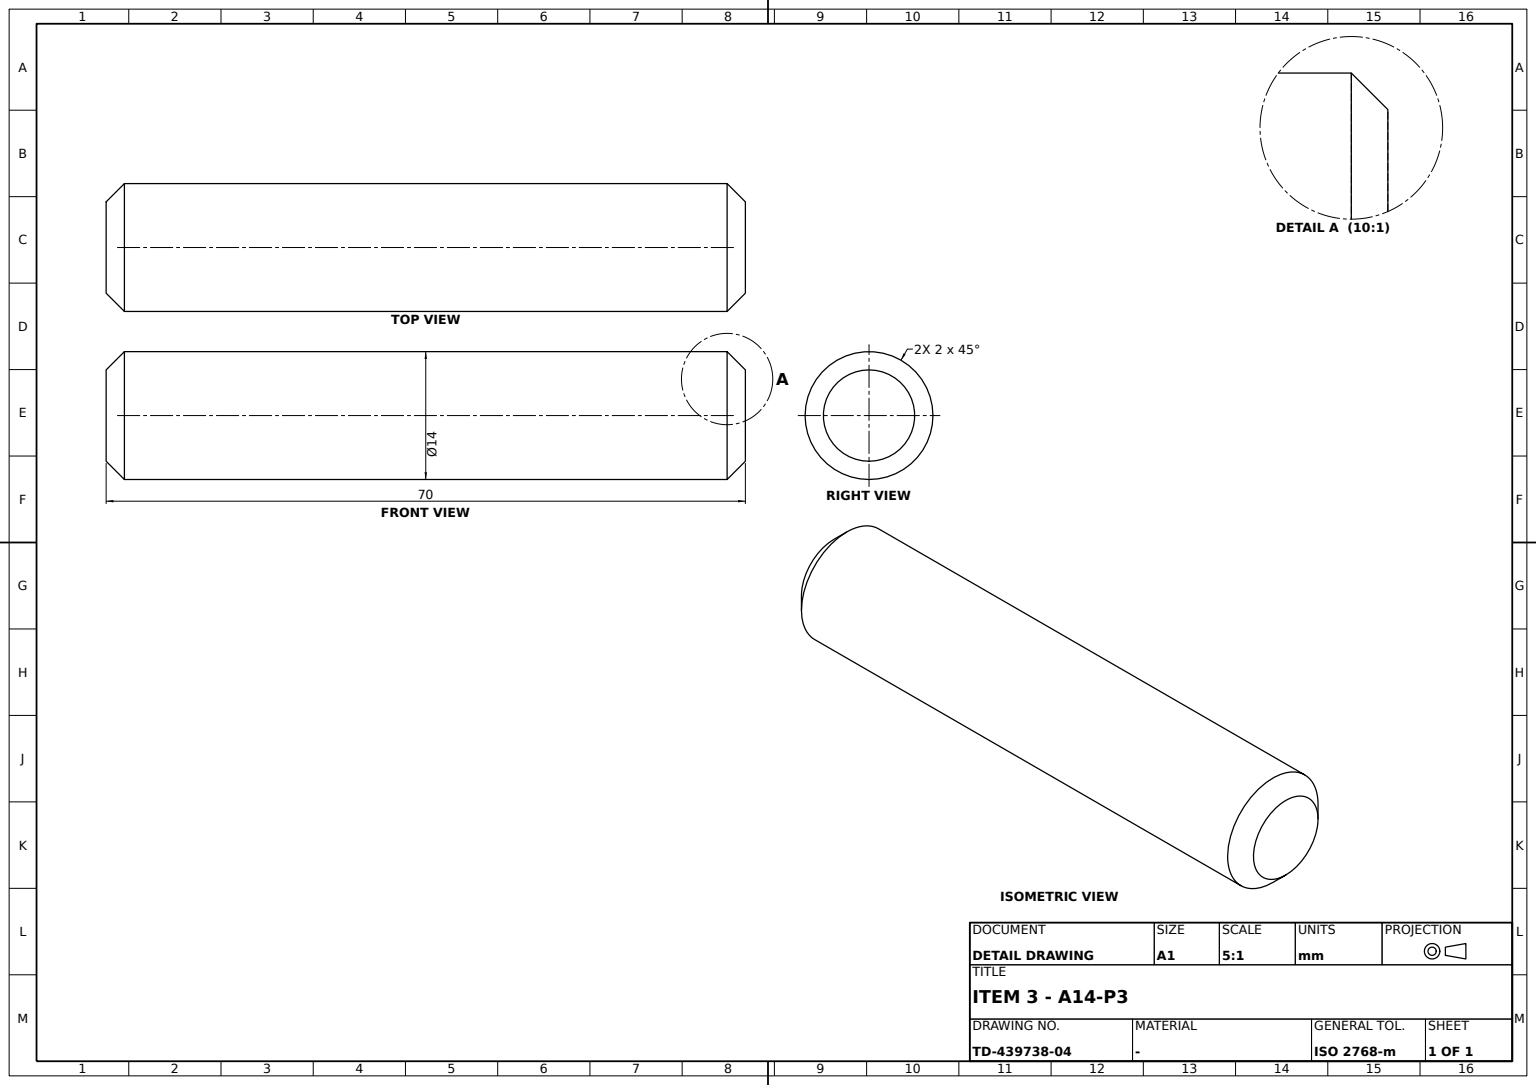
ISO-10303-21;
HEADER;
FILE_DESCRIPTION((''),'2;1');
FILE_NAME('','',(''),(''),'','','');
FILE_SCHEMA(('AUTOMOTIVE_DESIGN'));
ENDSEC;
DATA;
#1=APPLICATION_CONTEXT('');
#2=PRODUCT_CONTEXT('',#1,'mechanical');
#3=PRODUCT('','','',(#2));
#4=PRODUCT_DEFINITION_FORMATION('','',#3);
#5=PRODUCT_DEFINITION_CONTEXT('',#1,'design');
#6=PRODUCT_DEFINITION('','',#4,#5);
#7=PRODUCT_DEFINITION_SHAPE('','',#6);
#8=(LENGTH_UNIT()NAMED_UNIT(*)SI_UNIT(.MILLI.,.METRE.));
#9=(NAMED_UNIT(*)PLANE_ANGLE_UNIT()SI_UNIT($,.RADIAN.));
#10=(NAMED_UNIT(*)SI_UNIT($,.STERADIAN.)SOLID_ANGLE_UNIT());
#11=UNCERTAINTY_MEASURE_WITH_UNIT(LENGTH_MEASURE(0.005),#8,'distance_accuracy_value','');
#12=(GEOMETRIC_REPRESENTATION_CONTEXT(3)GLOBAL_UNCERTAINTY_ASSIGNED_CONTEXT((#11))GLOBAL_UNIT_ASSIGNED_CONTEXT((#8,#9,#10))REPRESENTATION_CONTEXT('',''));
#13=CARTESIAN_POINT('',(-2.,-7.,0.));
#14=VERTEX_POINT('',#13);
#15=CARTESIAN_POINT('',(-2.,0.,0.));
#16=DIRECTION('',(-1.,0.,0.));
#17=DIRECTION('',(0.,-1.,0.));
#18=AXIS2_PLACEMENT_3D('',#15,#16,#17);
#19=CIRCLE('',#18,7.);
#20=EDGE_CURVE('',#14,#14,#19,.F.);
#21=ORIENTED_EDGE('',*,*,#20,.T.);
#22=EDGE_LOOP('',(#21));
#23=FACE_BOUND('',#22,.T.);
#24=CARTESIAN_POINT('',(0.,0.,-5.));
#25=VERTEX_POINT('',#24);
#26=CARTESIAN_POINT('',(0.,0.,0.));
#27=DIRECTION('',(1.,0.,0.));
#28=DIRECTION('',(0.,0.,-1.));
#29=AXIS2_PLACEMENT_3D('',#26,#27,#28);
#30=CIRCLE('',#29,5.);
#31=EDGE_CURVE('',#25,#25,#30,.T.);
#32=ORIENTED_EDGE('',*,*,#31,.F.);
#33=EDGE_LOOP('',(#32));
#34=FACE_BOUND('',#33,.T.);
#35=CARTESIAN_POINT('',(5.,0.,0.));
#36=DIRECTION('',(0.,0.5,-0.866025404));
#37=AXIS2_PLACEMENT_3D('',#35,#16,#36);
#38=CONICAL_SURFACE('',#37,0.,0.785398163);
#39=ADVANCED_FACE('',(#23,#34),#38,.T.);
#40=CARTESIAN_POINT('',(-70.,0.,-5.));
#41=VERTEX_POINT('',#40);
#42=CARTESIAN_POINT('',(-70.,0.,0.));
#43=AXIS2_PLACEMENT_3D('',#42,#27,#28);
#44=CIRCLE('',#43,5.);
#45=EDGE_CURVE('',#41,#41,#44,.T.);
#46=ORIENTED_EDGE('',*,*,#45,.F.);
#47=EDGE_LOOP('',(#46));
#48=FACE_BOUND('',#47,.T.);
#49=DIRECTION('',(0.,1.,0.));
#50=AXIS2_PLACEMENT_3D('',#42,#27,#49);
#51=PLANE('',#50);
#52=ADVANCED_FACE('',(#48),#51,.F.);
#53=ORIENTED_EDGE('',*,*,#31,.T.);
#54=EDGE_LOOP('',(#53));
#55=FACE_BOUND('',#54,.T.);
#56=AXIS2_PLACEMENT_3D('',#26,#27,#49);
#57=PLANE('',#56);
#58=ADVANCED_FACE('',(#55),#57,.T.);
#59=ORIENTED_EDGE('',*,*,#45,.T.);
#60=EDGE_LOOP('',(#59));
#61=FACE_BOUND('',#60,.T.);
#62=CARTESIAN_POINT('',(-68.,7.,0.));
#63=VERTEX_POINT('',#62);
#64=CARTESIAN_POINT('',(-68.,0.,0.));
#65=AXIS2_PLACEMENT_3D('',#64,#27,#49);
#66=CIRCLE('',#65,7.);
#67=EDGE_CURVE('',#63,#63,#66,.T.);
#68=ORIENTED_EDGE('',*,*,#67,.F.);
#69=EDGE_LOOP('',(#68));
#70=FACE_BOUND('',#69,.T.);
#71=CARTESIAN_POINT('',(-75.,0.,0.));
#72=DIRECTION('',(0.,-0.5,0.866025404));
#73=AXIS2_PLACEMENT_3D('',#71,#27,#72);
#74=CONICAL_SURFACE('',#73,0.,0.785398163);
#75=ADVANCED_FACE('',(#61,#70),#74,.T.);
#76=ORIENTED_EDGE('',*,*,#67,.T.);
#77=EDGE_LOOP('',(#76));
#78=FACE_BOUND('',#77,.T.);
#79=ORIENTED_EDGE('',*,*,#20,.F.);
#80=EDGE_LOOP('',(#79));
#81=FACE_BOUND('',#80,.T.);
#82=CARTESIAN_POINT('',(-35.,0.,0.));
#83=AXIS2_PLACEMENT_3D('',#82,#27,#49);
#84=CYLINDRICAL_SURFACE('',#83,7.);
#85=ADVANCED_FACE('',(#78,#81),#84,.T.);
#86=CLOSED_SHELL('',(#39,#52,#58,#75,#85));
#87=MANIFOLD_SOLID_BREP('',#86);
#88=ADVANCED_BREP_SHAPE_REPRESENTATION('',(#87),#12);
#89=SHAPE_DEFINITION_REPRESENTATION(#7,#88);
ENDSEC;
END-ISO-10303-21;
